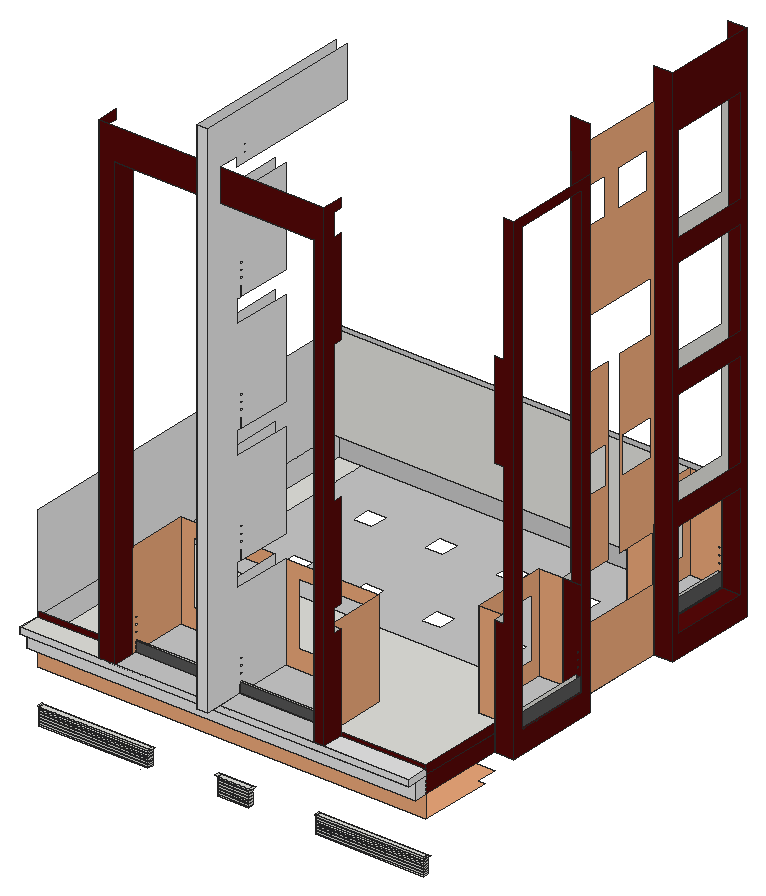
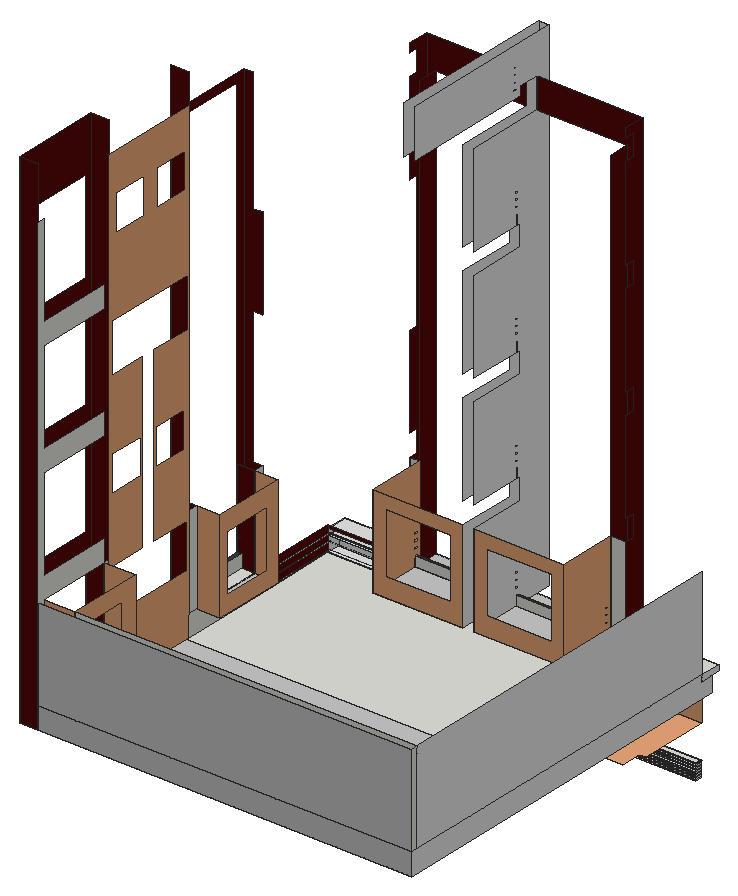
# SketchUp Ruby script. Lengths in inches.
U = 1.inch
M = Sketchup.active_model
def pt(a) = Geom::Point3d.new(a.map { |v| v * U })
def face(e, loops, mat)
  f = e.add_face(loops[0].map { |a| pt(a) })
  loops[1..].each { |l| e.add_face(l.map { |a| pt(a) }).erase! }
  f.material = f.back_material = mat if mat
  f
end
# faces: each face lists its corners as indices into pts; further lists are holes
def faces(e, pts, list, mat = nil) = list.each { |f| face(e, (f[0].is_a?(Array) ? f : [f]).map { |l| l.map { |i| pts[i] } }, mat) }
# xy, xz, yz: faces in a plane at the given z, y or x. An outline is a flat list of corners, or four numbers for a rectangle; further outlines are holes
def ring(l) = l.size == 4 ? [[l[0], l[1]], [l[2], l[1]], [l[2], l[3]], [l[0], l[3]]] : l.each_slice(2).to_a
def flat(e, list, mat, &to3) = list.each { |f| face(e, (f[0].is_a?(Array) ? f : [f]).map { |l| ring(l).map { |u, v| to3.(u, v) } }, mat) }
def xy(e, z, list, mat = nil) = flat(e, list, mat) { |x, y| [x, y, z] }
def xz(e, y, list, mat = nil) = flat(e, list, mat) { |x, z| [x, y, z] }
def yz(e, x, list, mat = nil) = flat(e, list, mat) { |y, z| [x, y, z] }
def lines(e, pts, list) = list.each { |a, b| e.add_line(pt(pts[a]), pt(pts[b])) }
# prism: a flat outline (further loops are holes) pulled along v
def prism(e, loops, v, mat = nil)
  f = face(e, loops, mat); d = Geom::Vector3d.new(v.map { |x| x * U })
  f.pushpull(f.normal.samedirection?(d) ? d.length : -d.length)
end
def box(e, o, s, mat = nil) = prism(e, [[o, [o[0] + s[0], o[1], o[2]], [o[0] + s[0], o[1] + s[1], o[2]], [o[0], o[1] + s[1], o[2]]]], [0, 0, s[2]], mat)
def at(x, y, z, deg = 0) = Geom::Transformation.translation(pt([x, y, z])) * Geom::Transformation.rotation(ORIGIN, Z_AXIS, deg.degrees)
def axes(o, x, y, z) = Geom::Transformation.new([*x, 0, *y, 0, *z, 0, *pt(o).to_a, 1])
def part(name) = M.definitions.add(name)
# library, detail: a bought-in or finely detailed component or shape, given as its bounding box
def library(name, o, s) = part(name).tap { |d| box(d.entities, o, s) }
def detail(e, o, s) = box(e.add_group.entities, o, s)
def put(e, d, t, mat = nil) = e.add_instance(d, t).tap { |i| i.material = mat if mat }
def group(e, t, mat = nil) = e.add_group.tap { |g| g.transformation = t; g.material = mat if mat }.entities
root = M.entities
M.materials.add("Generic").color = [86, 8, 8]
M.materials.add("Generic\#1").color = [236, 168, 122]
M.materials.add("Generic\#4").color = [201, 201, 201]
M.materials.add("Generic\#5").color = [230, 230, 230]
M.materials.add("[Color M06]").color = [86, 86, 86]
xy(root,37.0625,[[19.375,113.625,211.0625,122.8125],[332.7,113.625,387.73,122.8125],[505.65,113.625,694.3125,122.8125]])
xy(root,39.0625,[[19.375,113.625,211.0625,122.8125],[332.7,113.625,387.73,122.8125],[505.65,113.625,694.3125,122.8125]])
xy(root,42.0625,[[19.375,113.625,211.0625,122.8125],[332.7,113.625,387.73,122.8125],[505.65,113.625,694.3125,122.8125]])
xy(root,44.0625,[[19.375,113.625,211.0625,122.8125],[332.7,113.625,387.73,122.8125],[505.65,113.625,694.3125,122.8125]])
xy(root,47.0625,[[19.375,113.625,211.0625,122.8125],[332.7,113.625,387.73,122.8125],[505.65,113.625,694.3125,122.8125]])
xy(root,49.0625,[[19.375,113.625,211.0625,122.8125],[332.7,113.625,387.73,122.8125],[505.65,113.625,694.3125,122.8125]])
xy(root,52.0625,[[19.375,113.625,211.0625,122.8125],[332.7,113.625,387.73,122.8125],[505.65,113.625,694.3125,122.8125]])
xy(root,54.0625,[[19.375,113.625,211.0625,122.8125],[332.7,113.625,387.73,122.8125],[505.65,113.625,694.3125,122.8125]])
xy(root,57.0625,[[19.375,113.625,211.0625,122.8125],[332.7,113.625,387.73,122.8125],[505.65,113.625,694.3125,122.8125]])
xy(root,59.0625,[[19.375,113.625,211.0625,122.8125],[332.7,113.625,387.73,122.8125],[505.65,113.625,694.3125,122.8125]])
xy(root,62.0625,[[19.375,113.625,211.0625,122.8125],[332.7,113.625,387.73,122.8125],[505.65,113.625,694.3125,122.8125]])
xy(root,64.0625,[[19.375,113.625,211.0625,122.8125],[505.5625,113.625,694.3125,122.8125]])
xy(root,67.0625,[[16.6875,113.625,19.375,122.8125],[19.375,113.625,211.0625,122.8125],[211.0625,113.625,215.625,122.8125],[327,113.625,332.7,122.8125],[332.7,113.625,387.61,122.8125],
  [387.61,113.625,391.97,122.8125],[502.82,113.625,505.5625,122.8125],[505.5625,113.625,505.65,122.8125],[505.65,113.625,694.3125,122.8125],[694.3125,113.625,698.4375,122.8125]])
xy(root,128.3125,[[16.6875,113.625,16.6875,241.3125,28.6875,241.3125,28.6875,278.75,175.125,278.75,175.125,241.3125,187.125,241.3125,187.125,278.75,345.5625,278.75,345.5625,241.3125,357.5625,241.3125,357.5625,278.75,516,278.75,516,241.3125,528,241.3125,528,278.75,686.4375,278.75,686.4375,241.3125,698.4375,241.3125,698.4375,113.625]],"Generic\#1")
xy(root,168,[[16.6875,113.625,16.6875,774.8125,56.125,774.8125,56.125,437.0625,698.4375,437.0625,698.4375,113.625]])
xy(root,168,[[698.4375,263.625,731.4375,431.625],[698.4375,612.8125,731.4375,774.8125]],"Generic")
xy(root,168,[[[56.125,437.0625,698.4375,774.8125],[640.76,649.6,674.95,683.79],[515.63,649.6,549.82,683.79],[390.51,649.6,424.7,683.79],[265.38,649.6,299.57,683.79],[140.26,649.6,174.45,683.79],[140.26,487.6,174.45,521.79],[265.38,487.6,299.57,521.79],[390.51,487.6,424.7,521.79],[515.63,487.6,549.82,521.79],[640.76,487.6,674.95,521.79]]],"Generic\#4")
xy(root,168,[[16.6875,89.9375,698.4375,113.625]],"Generic\#5")
xy(root,196.375,[[16.6875,89.9375,698.4375,113.625]])
xy(root,196.375,[[16.6875,75.4375,698.4375,89.9375]],"Generic\#5")
xy(root,197.3125,[[698.14,113.625,698.4375,263.625]])
xy(root,198.3125,[[698.14,113.625,698.4375,263.625]])
xy(root,204.875,[[367.1875,119.625,531.5625,123.625]])
xy(root,207.3125,[[347.9375,48.1875,367.1875,75.4375],[16.6875,75.4375,154.5,113.625],[154.5,75.4375,183.4375,113.625],[183.4375,75.4375,183.5625,113.625],[347.9375,75.4375,367.1875,113.625],
  [531.5625,75.4375,531.6875,113.625],[531.6875,75.4375,549.5625,113.625],[183.5625,119.625,347.9375,123.625],[367.1875,119.625,531.5625,123.625],[698.4375,281.625,721.6875,413.625],
  [691.25,624.8125,695.75,762.8125],[695.75,624.8125,698.4375,762.8125]])
xy(root,207.3125,[[728.4375,281.625,731.4375,413.625],[698.4375,624.8125,731.4375,762.8125]],"Generic")
xy(root,207.3125,[[183.5625,75.4375,347.9375,119.625],[367.1875,75.4375,531.5625,119.625],[183.5625,123.625,347.9375,219.4375],[367.1875,123.625,531.5625,219.4375],[656.0625,281.625,698.4375,413.625],
  [641.125,624.8125,691.25,762.8125]],"Generic\#4")
xy(root,207.3125,[[549.5625,75.4375,698.4375,113.625]],"Generic\#5")
xz(root,48.1875,[[347.9375,207.3125,367.1875,1124.875]],"Generic\#5")
xz(root,75.4375,[[154.5,207.3125,183.4375,207.3125,183.4375,997.25,347.9375,997.25,347.9375,1052.9375,154.5,1052.9375],[531.6875,207.3125,549.5625,207.3125,549.5625,1052.9375,367.1875,1052.9375,367.1875,997.25,531.6875,997.25]],"Generic")
xz(root,75.4375,[[16.6875,196.375,698.4375,207.3125]],"Generic\#5")
xz(root,89.9375,[[16.6875,168,698.4375,196.375]],"Generic\#5")
xz(root,113.625,[[19.375,39.0625,211.0625,42.0625],[332.7,39.0625,387.61,42.0625],[387.61,39.0625,387.73,42.0625],[505.65,39.0625,694.3125,42.0625],[19.375,44.0625,211.0625,47.0625],
  [332.7,44.0625,387.61,47.0625],[387.61,44.0625,387.73,47.0625],[505.65,44.0625,694.3125,47.0625],[19.375,49.0625,211.0625,52.0625],[332.7,49.0625,387.61,52.0625],
  [387.61,49.0625,387.73,52.0625],[505.65,49.0625,694.3125,52.0625],[19.375,54.0625,211.0625,57.0625],[332.7,54.0625,387.61,57.0625],[387.61,54.0625,387.73,57.0625],
  [505.65,54.0625,694.3125,57.0625],[19.375,59.0625,211.0625,62.0625],[332.7,59.0625,387.61,62.0625],[387.61,59.0625,387.73,62.0625],[505.65,59.0625,694.3125,62.0625],
  [19.375,64.0625,211.0625,67.0625],[332.7,64.0625,387.61,67.0625],[505.5625,64.0625,505.65,67.0625],[505.65,64.0625,694.3125,67.0625],[698.14,169.8125,698.4375,170.8125],
  [698.14,183.5625,698.4375,184.5625],[549.5625,186,698.4375,187],[698.14,197.3125,698.4375,198.3125],[549.5625,199.5625,698.4375,200.5625],[154.5,207.3125,183.4375,375.3125],
  [183.4375,207.3125,183.5625,375.3125],[531.5625,207.3125,531.6875,375.3125],[531.6875,207.3125,549.5625,375.3125]])
xz(root,113.625,[[16.6875,207.3125,154.5,217],[549.5625,207.3125,698.4375,213.125]],"Generic")
xz(root,113.625,[[16.6875,128.3125,698.4375,168]],"Generic\#1")
xz(root,119.625,[[367.1875,204.875,531.5625,207.3125]])
xz(root,119.625,[[183.5625,207.3125,347.9375,225.3125],[367.1875,207.3125,531.5625,225.3125]],"[Color M06]")
xz(root,122.8125,[[19.375,39.0625,211.0625,42.0625],[332.7,39.0625,387.61,42.0625],[387.61,39.0625,387.73,42.0625],[505.65,39.0625,694.3125,42.0625],[19.375,44.0625,211.0625,47.0625],
  [332.7,44.0625,387.61,47.0625],[387.61,44.0625,387.73,47.0625],[505.65,44.0625,694.3125,47.0625],[19.375,49.0625,211.0625,52.0625],[332.7,49.0625,387.61,52.0625],
  [387.61,49.0625,387.73,52.0625],[505.65,49.0625,694.3125,52.0625],[19.375,54.0625,211.0625,57.0625],[332.7,54.0625,387.61,57.0625],[387.61,54.0625,387.73,57.0625],
  [505.65,54.0625,694.3125,57.0625],[19.375,59.0625,211.0625,62.0625],[332.7,59.0625,387.61,62.0625],[387.61,59.0625,387.73,62.0625],[505.65,59.0625,694.3125,62.0625],
  [19.375,64.0625,211.0625,67.0625],[332.7,64.0625,387.61,67.0625],[505.5625,64.0625,505.65,67.0625],[505.65,64.0625,694.3125,67.0625]])
xz(root,123.625,[[367.1875,204.875,531.5625,207.3125],[183.5625,207.3125,347.9375,225.3125],[367.1875,207.3125,531.5625,225.3125]])
xz(root,219.4375,[[[183.5625,207.3125,347.9375,375.3125],[205.67,241.4,323.42,351.52]],[[367.1875,207.3125,531.5625,375.3125],[390.3,241.4,508.05,351.52]]],"Generic\#1")
xz(root,263.625,[[698.14,169.8125,698.4375,170.8125],[698.14,183.5625,698.4375,184.5625],[698.14,197.3125,698.4375,198.3125]])
xz(root,263.625,[[698.4375,168,731.4375,168,731.4375,1012.8125,715.125,1012.8125,715.125,789.9375,698.4375,789.9375,698.4375,621.9375,715.125,621.9375,715.125,375.3125,698.4375,375.3125]],"Generic")
xz(root,281.625,[[[698.4375,207.3125,698.4375,375.3125,731.4375,375.3125,731.4375,207.3125,728.4375,207.3125,728.4375,231.3125,721.6875,231.3125,721.6875,207.3125],[722.9,266.36,726.28,269.49],[722.9,254.55,726.28,257.67],[722.9,242.55,726.28,245.67]]],"Generic")
xz(root,281.625,[[656.0625,207.3125,698.4375,375.3125]],"Generic\#1")
xz(root,413.625,[[[698.4375,207.3125,721.6875,207.3125,721.6875,231.3125,728.4375,231.3125,728.4375,207.3125,731.4375,207.3125,731.4375,375.3125,698.4375,375.3125],[722.9,266.36,726.28,269.49],[722.9,254.55,726.28,257.67],[722.9,242.55,726.28,245.67]]],"Generic")
xz(root,413.625,[[656.0625,207.3125,698.4375,375.3125]],"Generic\#1")
xz(root,431.625,[[698.4375,168,698.4375,1093.1875,731.4375,1093.1875,731.4375,1081.1875,731.14,1081.1875,731.14,1080.1875,731.4375,1080.1875,731.4375,1071.5625,731.14,1071.5625,731.14,1070.5625,731.4375,1070.5625,731.4375,1061.9375,731.14,1061.9375,731.14,1060.9375,731.4375,1060.9375,731.4375,1052.3125,731.14,1052.3125,731.14,1051.3125,731.4375,1051.3125,731.4375,1042.6875,731.14,1042.6875,731.14,1041.6875,731.4375,1041.6875,731.4375,1033.0625,731.14,1033.0625,731.14,1032.0625,731.4375,1032.0625,731.4375,1023.4375,731.14,1023.4375,731.14,1022.4375,731.4375,1022.4375,731.4375,1013.8125,731.14,1013.8125,731.14,1012.8125,731.4375,1012.8125,731.4375,168]],"Generic")
xz(root,612.8125,[[698.4375,168,731.4375,1093.1875]],"Generic")
xz(root,624.8125,[[691.25,207.3125,695.75,231.3125]])
xz(root,624.8125,[[698.4375,207.3125,731.4375,375.3125]],"Generic")
xz(root,624.8125,[[[641.125,207.3125,641.125,375.3125,698.4375,375.3125,698.4375,207.3125,695.75,207.3125,695.75,231.3125,691.25,231.3125,691.25,207.3125],[691.43,266.42,695.61,269.74],[691.43,254.42,695.61,257.74],[691.43,242.42,695.61,245.74]]],"Generic\#1")
xz(root,762.8125,[[16.6875,207.3125,641.125,375.3125],[691.25,207.3125,695.75,231.3125]])
xz(root,762.8125,[[698.4375,207.3125,731.4375,375.3125]],"Generic")
xz(root,762.8125,[[[641.125,207.3125,691.25,207.3125,691.25,231.3125,695.75,231.3125,695.75,207.3125,698.4375,207.3125,698.4375,375.3125,641.125,375.3125],[691.43,266.42,695.61,269.74],[691.43,254.42,695.61,257.74],[691.43,242.42,695.61,245.74]]],"Generic\#1")
xz(root,774.8125,[[698.4375,168,731.4375,1093.1875]],"Generic")
xz(root,774.8125,[[16.6875,168,698.4375,207.3125],[16.6875,207.3125,698.4375,375.3125]],"Generic\#4")
yz(root,16.6875,[[762.8125,207.3125,774.8125,375.3125]])
yz(root,16.6875,[[89.9375,168,89.9375,196.375,113.625,196.375,113.625,207.3125,774.8125,207.3125,774.8125,168],[75.4375,196.375,113.625,207.3125],[113.625,207.3125,113.625,217,113.92,217,113.92,218,113.625,218,113.625,226.6875,113.92,226.6875,113.92,227.6875,113.625,227.6875,113.625,236.375,113.92,236.375,113.92,237.375,113.625,237.375,113.625,246.0625,113.92,246.0625,113.92,247.0625,113.625,247.0625,113.625,255.75,113.92,255.75,113.92,256.75,113.625,256.75,113.625,265.4375,113.92,265.4375,113.92,266.4375,113.625,266.4375,113.625,275.125,113.92,275.125,113.92,276.125,113.625,276.125,113.625,284.8125,113.92,284.8125,113.92,285.8125,113.625,285.8125,113.625,294.5,113.92,294.5,113.92,295.5,113.625,295.5,113.625,304.1875,113.92,304.1875,113.92,305.1875,113.625,305.1875,113.625,313.875,113.92,313.875,113.92,314.875,113.625,314.875,113.625,323.5625,113.92,323.5625,113.92,324.5625,113.625,324.5625,113.625,333.25,113.92,333.25,113.92,334.25,113.625,334.25,113.625,342.9375,113.92,342.9375,113.92,343.9375,113.625,343.9375,113.625,352.625,113.92,352.625,113.92,353.625,113.625,353.625,113.625,362.3125,113.92,362.3125,113.92,363.3125,113.625,363.3125,113.625,375.3125,762.8125,375.3125,762.8125,207.3125]],"Generic\#5")
yz(root,19.375,[[113.625,37.0625,122.8125,39.0625],[113.625,39.0625,122.8125,42.0625],[113.625,42.0625,122.8125,44.0625],[113.625,44.0625,122.8125,47.0625],[113.625,47.0625,122.8125,49.0625],
  [113.625,49.0625,122.8125,52.0625],[113.625,52.0625,122.8125,54.0625],[113.625,54.0625,122.8125,57.0625],[113.625,57.0625,122.8125,59.0625],[113.625,59.0625,122.8125,62.0625],
  [113.625,62.0625,122.8125,64.0625],[113.625,64.0625,122.8125,67.0625]])
yz(root,154.5,[[75.4375,207.3125,75.4375,1052.9375,113.625,1052.9375,113.625,1036.5625,96.5625,1036.5625,96.5625,997.25,113.625,997.25,113.625,829.25,96.5625,829.25,96.5625,789.9375,113.625,789.9375,113.625,621.9375,96.5625,621.9375,96.5625,582.625,113.625,582.625,113.625,414.625,96.5625,414.625,96.5625,375.3125,113.625,375.3125,113.625,207.3125]],"Generic")
yz(root,183.4375,[[75.4375,207.3125,113.625,997.25]],"Generic")
yz(root,183.5625,[[119.625,207.3125,123.625,225.3125]])
yz(root,183.5625,[[[113.625,207.3125,119.625,207.3125,119.625,225.3125,123.625,225.3125,123.625,207.3125,219.4375,207.3125,219.4375,375.3125,113.625,375.3125],[118.5,259.82,125.9375,263.63],[118.5,247.82,125.9375,251.63],[118.5,235.82,125.9375,239.63]]],"Generic\#1")
yz(root,211.0625,[[113.625,37.0625,122.8125,39.0625],[113.625,39.0625,122.8125,42.0625],[113.625,42.0625,122.8125,44.0625],[113.625,44.0625,122.8125,47.0625],[113.625,47.0625,122.8125,49.0625],
  [113.625,49.0625,122.8125,52.0625],[113.625,52.0625,122.8125,54.0625],[113.625,54.0625,122.8125,57.0625],[113.625,57.0625,122.8125,59.0625],[113.625,59.0625,122.8125,62.0625],
  [113.625,62.0625,122.8125,64.0625]])
yz(root,332.7,[[113.625,37.0625,122.8125,39.0625],[113.625,39.0625,122.8125,42.0625],[113.625,42.0625,122.8125,44.0625],[113.625,44.0625,122.8125,47.0625],[113.625,47.0625,122.8125,49.0625],
  [113.625,49.0625,122.8125,52.0625],[113.625,52.0625,122.8125,54.0625],[113.625,54.0625,122.8125,57.0625],[113.625,57.0625,122.8125,59.0625],[113.625,59.0625,122.8125,62.0625],
  [113.625,64.0625,122.8125,67.0625]])
yz(root,347.9375,[[119.625,207.3125,123.625,225.3125]])
yz(root,347.9375,[[[48.1875,207.3125,48.1875,1124.875,354.125,1124.875,354.125,1036.5625,113.625,1036.5625,113.625,1052.9375,75.4375,1052.9375,75.4375,997.25,219.4375,997.25,219.4375,829.25,123.625,829.25,123.625,847.25,119.625,847.25,119.625,829.25,113.625,829.25,113.625,789.9375,219.4375,789.9375,219.4375,621.9375,123.625,621.9375,123.625,639.9375,119.625,639.9375,119.625,621.9375,113.625,621.9375,113.625,582.625,219.4375,582.625,219.4375,414.625,123.625,414.625,123.625,432.625,119.625,432.625,119.625,414.625,113.625,414.625,113.625,375.3125,219.4375,375.3125,219.4375,207.3125,123.625,207.3125,123.625,225.3125,119.625,225.3125,119.625,207.3125],[118.5,235.82,125.9375,239.63],[118.5,247.82,125.9375,251.63],[118.5,259.82,125.9375,263.63],[118.5,442.38,125.9375,446.19],[118.5,454.38,125.9375,458.19],[118.5,466.73,125.9375,470.54],[118.5,650.73,125.9375,654.54],[118.5,662.73,125.9375,666.54],[118.5,674.73,125.9375,678.54],[118.5,857.85,125.9375,861.67],[118.5,869.85,125.9375,873.67],[118.5,880.92,125.9375,884.73],[122.52,1051.13,129.9,1053.13],[123.11,1063.19,128.18,1065.32],[123.11,1075.19,128.18,1077.32],[123.11,1087.19,128.18,1089.32]]],"Generic\#5")
yz(root,367.1875,[[119.625,204.875,123.625,207.3125],[119.625,207.3125,123.625,225.3125]])
yz(root,367.1875,[[[48.1875,207.3125,119.625,207.3125,119.625,225.3125,123.625,225.3125,123.625,207.3125,219.4375,207.3125,219.4375,375.3125,113.625,375.3125,113.625,414.625,119.625,414.625,119.625,432.625,123.625,432.625,123.625,414.625,219.4375,414.625,219.4375,582.625,113.625,582.625,113.625,621.9375,119.625,621.9375,119.625,639.9375,123.625,639.9375,123.625,621.9375,219.4375,621.9375,219.4375,789.9375,113.625,789.9375,113.625,829.25,119.625,829.25,119.625,847.25,123.625,847.25,123.625,829.25,219.4375,829.25,219.4375,997.25,75.4375,997.25,75.4375,1052.9375,113.625,1052.9375,113.625,1036.5625,354.125,1036.5625,354.125,1124.875,48.1875,1124.875],[118.5,235.82,125.9375,239.63],[118.5,247.82,125.9375,251.63],[118.5,259.82,125.9375,263.63],[118.5,442.82,125.9375,446.63],[118.5,454.82,125.9375,458.63],[118.5,466.82,125.9375,470.63],[118.5,650,125.9375,653.82],[118.5,662,125.9375,665.82],[118.5,674,125.9375,677.82],[118.5,857.82,125.9375,861.63],[118.5,869.58,125.9375,873.39],[118.5,881.34,125.9375,885.15],[126.95,1052.22,132.89,1055.1],[126.95,1064.22,132.89,1067.1],[126.95,1076.22,132.89,1079.1],[126.95,1087.4,132.89,1090.28]]],"Generic\#5")
yz(root,387.73,[[113.625,39.0625,122.8125,42.0625],[113.625,44.0625,122.8125,47.0625],[113.625,49.0625,122.8125,52.0625],[113.625,54.0625,122.8125,57.0625],[113.625,59.0625,122.8125,62.0625]])
yz(root,505.5625,[[113.625,64.0625,122.8125,67.0625]])
yz(root,505.65,[[113.625,37.0625,122.8125,39.0625],[113.625,39.0625,122.8125,42.0625],[113.625,42.0625,122.8125,44.0625],[113.625,44.0625,122.8125,47.0625],[113.625,47.0625,122.8125,49.0625],
  [113.625,49.0625,122.8125,52.0625],[113.625,52.0625,122.8125,54.0625],[113.625,54.0625,122.8125,57.0625],[113.625,57.0625,122.8125,59.0625],[113.625,59.0625,122.8125,62.0625],
  [113.625,62.0625,122.8125,67.0625]])
yz(root,531.5625,[[119.625,204.875,123.625,207.3125],[119.625,207.3125,123.625,225.3125]])
yz(root,531.5625,[[[113.625,207.3125,113.625,375.3125,219.4375,375.3125,219.4375,207.3125,123.625,207.3125,123.625,225.3125,119.625,225.3125,119.625,207.3125],[118.5,259.82,125.9375,263.63],[118.5,247.82,125.9375,251.63],[118.5,235.82,125.9375,239.63]]],"Generic\#1")
yz(root,531.6875,[[75.4375,207.3125,113.625,997.25]],"Generic")
yz(root,549.5625,[[75.4375,207.3125,113.625,207.3125,113.625,375.3125,96.5625,375.3125,96.5625,414.625,113.625,414.625,113.625,582.625,96.5625,582.625,96.5625,829.25,113.625,829.25,113.625,997.25,96.5625,997.25,96.5625,1036.5625,113.625,1036.5625,113.625,1052.9375,75.4375,1052.9375]],"Generic")
yz(root,641.125,[[[624.8125,207.3125,762.8125,375.3125],[655.17,241.63,747.23,344.94]]],"Generic\#1")
yz(root,656.0625,[[[281.625,207.3125,413.625,375.3125],[306.16,237.48,398.23,340.79]]],"Generic\#1")
yz(root,691.25,[[624.8125,207.3125,762.8125,231.3125]])
yz(root,694.3125,[[113.625,37.0625,122.8125,39.0625],[113.625,39.0625,122.8125,42.0625],[113.625,42.0625,122.8125,44.0625],[113.625,44.0625,122.8125,47.0625],[113.625,47.0625,122.8125,49.0625],
  [113.625,49.0625,122.8125,52.0625],[113.625,52.0625,122.8125,54.0625],[113.625,54.0625,122.8125,57.0625],[113.625,57.0625,122.8125,59.0625],[113.625,59.0625,122.8125,62.0625],
  [113.625,62.0625,122.8125,64.0625],[113.625,64.0625,122.8125,67.0625]])
yz(root,695.75,[[624.8125,207.3125,762.8125,231.3125]],"[Color M06]")
yz(root,698.14,[[113.625,169.8125,263.625,170.8125],[113.625,183.5625,263.625,184.5625],[113.625,197.3125,263.625,198.3125]])
yz(root,698.4375,[[263.625,168,431.625,207.3125],[612.8125,168,612.8125,207.3125,762.8125,207.3125,762.8125,375.3125,624.8125,375.3125,624.8125,414.625,762.8125,414.625,762.8125,582.625,624.8125,582.625,624.8125,621.9375,762.8125,621.9375,762.8125,789.9375,624.8125,789.9375,624.8125,829.25,762.8125,829.25,762.8125,997.25,774.8125,997.25,774.8125,168],[263.625,207.3125,281.625,375.3125],[413.625,207.3125,431.625,375.3125],[612.8125,207.3125,624.8125,375.3125]])
yz(root,698.4375,[[113.625,168,263.625,197.3125],[113.625,198.3125,263.625,213.125]],"Generic")
yz(root,698.4375,[[[431.625,168,612.8125,1036.5625],[436.65,279.02,436.65,361.33,510.93,361.33,510.93,672.98,434.68,672.98,434.68,762.91,606.05,762.91,606.05,672.98,537.45,672.98,537.45,361.33,610.59,361.33,610.59,279.02],[439.75,902.74,504.55,967.55],[533.62,902.74,598.43,967.55],[541.56,480.05,606.36,544.86],[441.62,480.05,506.43,544.86]]],"Generic\#1")
yz(root,698.4375,[[89.9375,168,113.625,196.375],[75.4375,196.375,113.625,207.3125]],"Generic\#5")
yz(root,721.6875,[[281.625,207.3125,413.625,231.3125]])
yz(root,728.4375,[[281.625,207.3125,413.625,231.3125]],"[Color M06]")
yz(root,731.4375,[[[263.625,168,431.625,1012.8125],[281.625,207.3125,413.625,997.25]],[612.8125,168,774.8125,168,774.8125,1093.1875,612.8125,1093.1875,612.8125,997.25,762.8125,997.25,762.8125,829.25,624.8125,829.25,624.8125,789.9375,762.8125,789.9375,762.8125,621.9375,624.8125,621.9375,624.8125,582.625,762.8125,582.625,762.8125,414.625,624.8125,414.625,624.8125,375.3125,762.8125,375.3125,762.8125,207.3125,624.8125,207.3125,624.8125,997.25,612.8125,997.25]],"Generic")
p = [[505.65,113.625,62.0625],[504.37,113.625,62.0625],[213.98,92.52,46.51],[213.98,92.52,46.125],[549.5625,113.625,173.4375],[698.4375,113.625,173.4375],
  [549.5625,113.625,172.4375],[549.5625,113.625,159.875],[549.5625,113.625,158.875]]
lines(root,p,[[0,1],[2,3],[4,5],[4,6],[7,8]])
